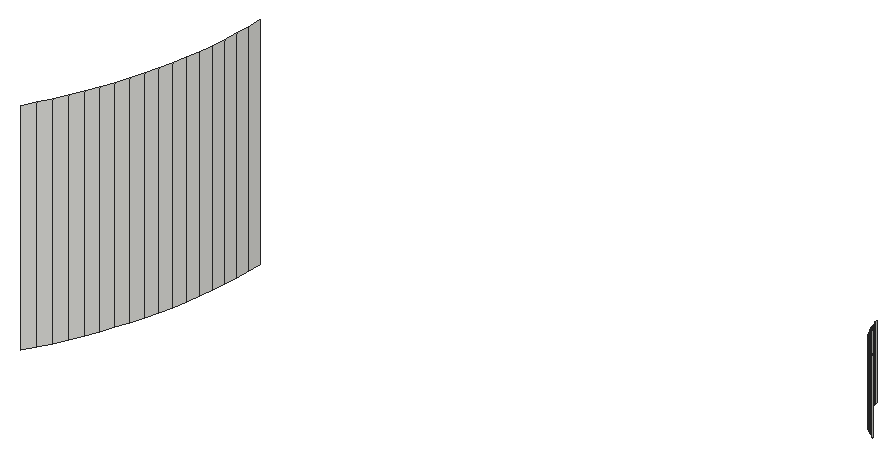
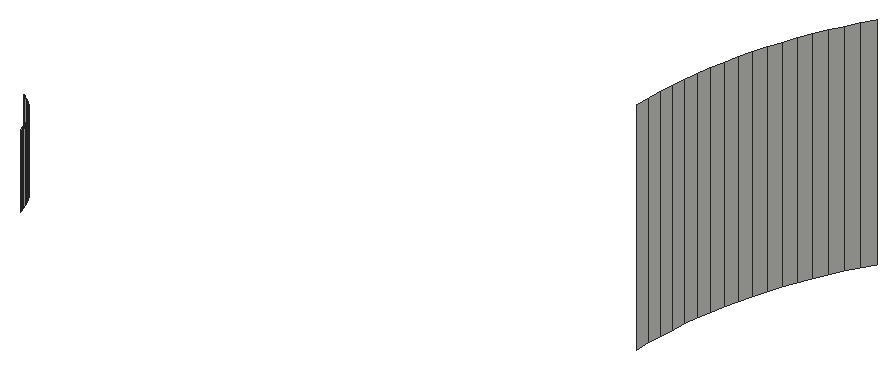
# SketchUp Ruby script. Lengths in inches.
U = 1.inch
M = Sketchup.active_model
def pt(a) = Geom::Point3d.new(a.map { |v| v * U })
def face(e, loops, mat)
  f = e.add_face(loops[0].map { |a| pt(a) })
  loops[1..].each { |l| e.add_face(l.map { |a| pt(a) }).erase! }
  f.material = f.back_material = mat if mat
  f
end
# faces: each face lists its corners as indices into pts; further lists are holes
def faces(e, pts, list, mat = nil) = list.each { |f| face(e, (f[0].is_a?(Array) ? f : [f]).map { |l| l.map { |i| pts[i] } }, mat) }
# xy, xz, yz: faces in a plane at the given z, y or x. An outline is a flat list of corners, or four numbers for a rectangle; further outlines are holes
def ring(l) = l.size == 4 ? [[l[0], l[1]], [l[2], l[1]], [l[2], l[3]], [l[0], l[3]]] : l.each_slice(2).to_a
def flat(e, list, mat, &to3) = list.each { |f| face(e, (f[0].is_a?(Array) ? f : [f]).map { |l| ring(l).map { |u, v| to3.(u, v) } }, mat) }
def xy(e, z, list, mat = nil) = flat(e, list, mat) { |x, y| [x, y, z] }
def xz(e, y, list, mat = nil) = flat(e, list, mat) { |x, z| [x, y, z] }
def yz(e, x, list, mat = nil) = flat(e, list, mat) { |y, z| [x, y, z] }
def lines(e, pts, list) = list.each { |a, b| e.add_line(pt(pts[a]), pt(pts[b])) }
# prism: a flat outline (further loops are holes) pulled along v
def prism(e, loops, v, mat = nil)
  f = face(e, loops, mat); d = Geom::Vector3d.new(v.map { |x| x * U })
  f.pushpull(f.normal.samedirection?(d) ? d.length : -d.length)
end
def box(e, o, s, mat = nil) = prism(e, [[o, [o[0] + s[0], o[1], o[2]], [o[0] + s[0], o[1] + s[1], o[2]], [o[0], o[1] + s[1], o[2]]]], [0, 0, s[2]], mat)
def at(x, y, z, deg = 0) = Geom::Transformation.translation(pt([x, y, z])) * Geom::Transformation.rotation(ORIGIN, Z_AXIS, deg.degrees)
def axes(o, x, y, z) = Geom::Transformation.new([*x, 0, *y, 0, *z, 0, *pt(o).to_a, 1])
def part(name) = M.definitions.add(name)
# library, detail: a bought-in or finely detailed component or shape, given as its bounding box
def library(name, o, s) = part(name).tap { |d| box(d.entities, o, s) }
def detail(e, o, s) = box(e.add_group.entities, o, s)
def put(e, d, t, mat = nil) = e.add_instance(d, t).tap { |i| i.material = mat if mat }
def group(e, t, mat = nil) = e.add_group.tap { |g| g.transformation = t; g.material = mat if mat }.entities
root = M.entities
p = [[156.49,236.84,357],[156.77,237.33,357],[156.77,237.33,348],[156.49,236.84,348],[157.04,237.83,357],[157.04,237.83,348],
  [157.29,238.34,357],[157.29,238.34,348],[157.52,238.85,357],[157.52,238.85,348],[157.74,239.375,357],[157.74,239.375,348],
  [157.9375,239.9,357],[157.9375,239.9,348],[158.12,240.4375,357],[158.12,240.4375,348],[158.29,240.98,357],[158.29,240.98,348],
  [158.43,241.52,357],[158.43,241.52,348],[158.57,242.07,357],[158.57,242.07,348],[158.68,242.63,357],[158.68,242.63,348],
  [158.78,243.18,357],[158.78,243.18,348],[158.86,243.74,357],[158.86,243.74,348],[158.92,244.31,357],[158.92,244.31,348],
  [158.96,244.87,357],[158.96,244.87,348],[158.99,245.43,357],[158.99,245.43,348],[159,246,357],[159,246,348],
  [181.43,249.44,348],[181.37,249.48,348],[181.37,249.48,351],[181.43,249.44,351],[181.3,249.53,348],[181.24,249.57,348],
  [181.24,249.57,351],[181.3,249.53,351],[181.17,249.62,348],[181.11,249.67,348],[181.11,249.67,351],[181.17,249.62,351],
  [181.05,249.72,348],[180.99,249.77,348],[180.99,249.77,351],[181.05,249.72,351],[180.93,249.82,348],[180.88,249.88,348],
  [180.88,249.88,351],[180.93,249.82,351],[180.82,249.94,348],[180.77,249.99,348],[180.77,249.99,351],[180.82,249.94,351],
  [180.72,250.05,348],[180.72,250.05,351],[180.67,250.11,348],[180.62,250.17,348],[180.62,250.17,351],[180.67,250.11,351],
  [180.57,250.24,348],[180.53,250.3,348],[180.53,250.3,351],[180.57,250.24,351],[180.48,250.37,348],[180.48,250.37,351],
  [180.44,250.43,348],[180.4,250.5,348],[180.4,250.5,351],[180.44,250.43,351],[180.36,250.57,348],[180.36,250.57,351],
  [180.33,250.64,348],[180.29,250.71,348],[180.29,250.71,351],[180.33,250.64,351],[180.26,250.78,348],[180.26,250.78,351],
  [180.23,250.85,348],[180.23,250.85,351],[180.2,250.93,348],[180.17,251,348],[180.17,251,351],[180.2,250.93,351],
  [180.15,251.07,348],[180.15,251.07,351],[180.125,251.15,348],[180.1,251.22,348],[180.1,251.22,351],[180.125,251.15,351],
  [180.08,251.3,348],[180.08,251.3,351]]
faces(root,p,[[0,1,2,3],[1,4,5,2],[4,6,7,5],[6,8,9,7],[8,10,11,9],[10,12,13,11],[12,14,15,13],[14,16,17,15],
  [16,18,19,17],[18,20,21,19],[20,22,23,21],[22,24,25,23],[24,26,27,25],[26,28,29,27],[28,30,31,29],[30,32,33,31],
  [32,34,35,33],[36,37,38,39],[40,41,42,43],[37,40,43,38],[44,45,46,47],[41,44,47,42],[48,49,50,51],[45,48,51,46],
  [52,53,54,55],[49,52,55,50],[56,57,58,59],[53,56,59,54],[57,60,61,58],[62,63,64,65],[60,62,65,61],[66,67,68,69],
  [63,66,69,64],[67,70,71,68],[72,73,74,75],[70,72,75,71],[73,76,77,74],[78,79,80,81],[76,78,81,77],[79,82,83,80],
  [82,84,85,83],[86,87,88,89],[84,86,89,85],[87,90,91,88],[92,93,94,95],[90,92,95,91],[93,96,97,94]])
